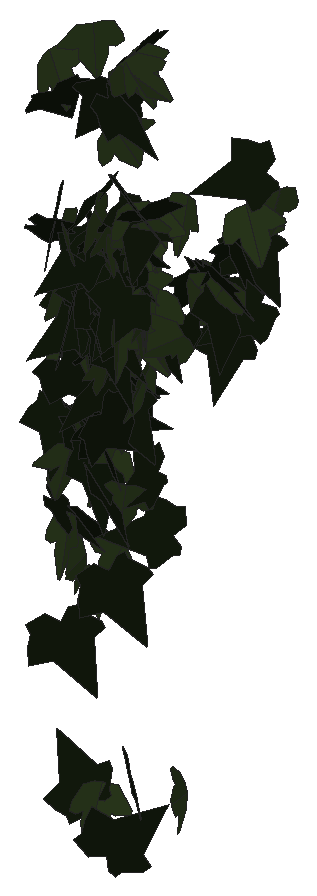
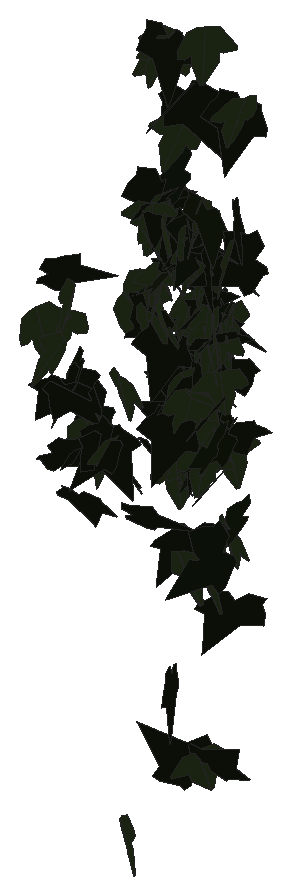
# SketchUp Ruby script. Lengths in inches.
U = 1.inch
M = Sketchup.active_model
def pt(a) = Geom::Point3d.new(a.map { |v| v * U })
def face(e, loops, mat)
  f = e.add_face(loops[0].map { |a| pt(a) })
  loops[1..].each { |l| e.add_face(l.map { |a| pt(a) }).erase! }
  f.material = f.back_material = mat if mat
  f
end
# faces: each face lists its corners as indices into pts; further lists are holes
def faces(e, pts, list, mat = nil) = list.each { |f| face(e, (f[0].is_a?(Array) ? f : [f]).map { |l| l.map { |i| pts[i] } }, mat) }
# xy, xz, yz: faces in a plane at the given z, y or x. An outline is a flat list of corners, or four numbers for a rectangle; further outlines are holes
def ring(l) = l.size == 4 ? [[l[0], l[1]], [l[2], l[1]], [l[2], l[3]], [l[0], l[3]]] : l.each_slice(2).to_a
def flat(e, list, mat, &to3) = list.each { |f| face(e, (f[0].is_a?(Array) ? f : [f]).map { |l| ring(l).map { |u, v| to3.(u, v) } }, mat) }
def xy(e, z, list, mat = nil) = flat(e, list, mat) { |x, y| [x, y, z] }
def xz(e, y, list, mat = nil) = flat(e, list, mat) { |x, z| [x, y, z] }
def yz(e, x, list, mat = nil) = flat(e, list, mat) { |y, z| [x, y, z] }
def lines(e, pts, list) = list.each { |a, b| e.add_line(pt(pts[a]), pt(pts[b])) }
# prism: a flat outline (further loops are holes) pulled along v
def prism(e, loops, v, mat = nil)
  f = face(e, loops, mat); d = Geom::Vector3d.new(v.map { |x| x * U })
  f.pushpull(f.normal.samedirection?(d) ? d.length : -d.length)
end
def box(e, o, s, mat = nil) = prism(e, [[o, [o[0] + s[0], o[1], o[2]], [o[0] + s[0], o[1] + s[1], o[2]], [o[0], o[1] + s[1], o[2]]]], [0, 0, s[2]], mat)
def at(x, y, z, deg = 0) = Geom::Transformation.translation(pt([x, y, z])) * Geom::Transformation.rotation(ORIGIN, Z_AXIS, deg.degrees)
def axes(o, x, y, z) = Geom::Transformation.new([*x, 0, *y, 0, *z, 0, *pt(o).to_a, 1])
def part(name) = M.definitions.add(name)
# library, detail: a bought-in or finely detailed component or shape, given as its bounding box
def library(name, o, s) = part(name).tap { |d| box(d.entities, o, s) }
def detail(e, o, s) = box(e.add_group.entities, o, s)
def put(e, d, t, mat = nil) = e.add_instance(d, t).tap { |i| i.material = mat if mat }
def group(e, t, mat = nil) = e.add_group.tap { |g| g.transformation = t; g.material = mat if mat }.entities
root = M.entities
M.materials.add("efeu1").color = [18, 25, 13]
M.materials.add("efeu2").color = [43, 57, 29]
c1 = part("ivyleaf_9")
p = [[1.54,2.16,1.25],[1.36,2.04,1.19],[-0.21,0.99,0.68],[-0.71,1.11,0.82],[-0.85,0.86,0.67],[-0.8,0.17,0.21],
  [-0.9,-0.01,0.1],[-0.67,-0.16,-0.02],[-0.08,-0.08,-0.05],[-0.03,-0.6,-0.4],[0.65,-0.88,-0.66],[0.83,-0.6,-0.49],
  [1.29,-0.42,-0.43],[1.8125,-0.07,-0.26],[1.21,0.44,0.15]]
faces(c1.entities,p,[[0,1,2,3,4,5,6,7,8,9,10,11,12,13,14]],"efeu1")
c2 = part("ivyleaf_10")
p = [[0,0.5,-0.03],[-0.0625,2.02,-0.43],[-0.19,2.01,-0.46],[-0.54,1.05,-0.29],[-0.52,0.625,-0.18],[-0.83,0.76,-0.28],
  [-1.16,0.64,-0.33],[-1.15,0.33,-0.24],[-0.77,-0.39,0.02],[-0.3,-0.51,0.16],[0.04,-0.48,0.23],[-0.02,2.01,-0.4375],
  [-0.06,2.01,-0.43],[0.04,-0.49,0.23],[0.67,-0.49,0.14],[1.38,0.36,-0.2],[1.375,0.51,-0.24],[0.81,0.65,-0.19],
  [0.62,0.59,-0.15],[0.6,1.09,-0.28],[0.5,1.23,-0.31]]
faces(c2.entities,p,[[0,1,2,3,4,5,6,7,8,9,10],[11,12,0,13,14,15,16,17,18,19,20]],"efeu2")
put(root,c1,axes([565.39,131.8,220.8125],[0.83802,-0.38885,-0.28194],[-0.1596,0.30932,-0.90101],[0.45302,0.8283,0.20411]))
put(root,c1,axes([565.19,131.24,232.89],[0.89104,0.08996,0.39688],[0.38144,0.14832,-0.88998],[-0.14182,0.96409,0.09988]))
put(root,c2,axes([565.66,139.23,230.36],[0.8859,-0.31674,0.10492],[0.10472,-0.01868,-0.94065],[0.3168,0.89189,0.01756]))
put(root,c2,axes([565.6875,131.4,240.08],[0.14938,0.96069,0.23258],[-0.00135,0.23542,-0.97155],[-0.98844,0.14487,0.03648]))
put(root,c2,axes([565.79,132.5,227.57],[0.61609,0.68863,-0.07239],[-0.08852,-0.01777,-0.92243],[-0.68675,0.62007,0.05396]))
put(root,c1,axes([565.35,133.52,225],[0.66113,-0.63323,0.0891],[0.06131,-0.0648,-0.91546],[0.63653,0.66395,-0.00436]))
put(root,c1,axes([565.79,131.85,224.875],[-0.50138,-0.7549,-0.20222],[0.13854,0.1506,-0.90569],[0.76914,-0.51922,0.03131]))
put(root,c1,axes([566.3125,139.5,227.53],[0.02633,0.74002,-0.55639],[-0.19435,-0.53979,-0.72715],[-0.90522,0.13742,0.13993]))
put(root,c2,axes([565.85,131.64,230.13],[0.23134,-0.92137,-0.0694],[0.23513,0.12789,-0.91412],[0.89357,0.20489,0.25851]))
put(root,c1,axes([565.45,133.04,219.62],[1.10906,-0.06823,0.04669],[0.0468,0.00039,-1.11115],[0.06816,1.11004,0.00326]))
put(root,c2,axes([566.0625,132.56,230.17],[0.3828,-0.85358,-0.16599],[0.00986,0.18561,-0.93173],[0.86951,0.37368,0.08364]))
put(root,c2,axes([566.08,132.49,229.6],[-0.87235,-0.34319,-0.15132],[0.14182,0.05284,-0.93743],[0.34722,-0.8838,0.00272]))
put(root,c2,axes([565.85,131.85,219.91],[0.87494,-0.39676,0.27622],[0.24314,-0.13251,-0.9605],[0.41785,0.90789,-0.01948]))
put(root,c1,axes([566.01,132.79,229.5],[-0.4877,-0.79464,-0.1327],[0.1525,0.06126,-0.92731],[0.79108,-0.5017,0.09695]))
put(root,c1,axes([565.7,133.05,223.02],[0.35096,-0.85963,-0.00658],[0.03008,0.01938,-0.92785],[0.85913,0.35049,0.03517]))
put(root,c2,axes([566.3,131.45,233.01],[-0.50537,0.74211,0.40736],[-0.25236,0.32079,-0.89749],[-0.80807,-0.5643,0.02552]))
put(root,c2,axes([566.26,132.27,224.74],[-0.32315,0.76023,0.42336],[-0.18241,0.3824,-0.8259],[-0.85083,-0.37072,0.01627]))
put(root,c1,axes([566.3,130.59,239.39],[0.35852,0.92403,-0.00446],[0.00246,-0.00573,-0.99114],[-0.92404,0.3585,-0.00437]))
put(root,c2,axes([566.15,139.51,227.28],[-0.11661,0.93037,0.21226],[-0.03849,0.20908,-0.93757],[-0.9535,-0.12223,0.01189]))
put(root,c1,axes([566.02,131.3,234.48],[-0.42055,0.14549,-0.8766],[0.80426,-0.35005,-0.44395],[-0.37783,-0.90706,0.03072]))
put(root,c1,axes([566.87,137.78,225.45],[-0.1541,0.45417,0.79811],[-0.45206,0.66689,-0.46678],[-0.7993,-0.46473,0.11013]))
put(root,c1,axes([566.92,131.92,208.59],[-0.95813,-0.20161,-0.2108],[-0.20468,-0.05099,0.97908],[-0.20782,0.97972,0.00758]))
put(root,c1,axes([565.86,132.18,224.74],[0.9116,-0.15725,-0.03229],[-0.02068,0.06961,-0.92277],[0.15919,0.90951,0.06504]))
put(root,c2,axes([566.5,131.22,223.54],[-0.32914,-0.89291,0.23218],[0.01638,-0.25213,-0.94641],[0.92245,-0.31412,0.09965]))
put(root,c1,axes([566.05,139.76,227.68],[0.91534,0.02089,-0.13093],[-0.13075,-0.00935,-0.91556],[-0.022,0.92461,-0.0063]))
put(root,c2,axes([566.47,132.9,223.89],[-0.6777,-0.63529,-0.08735],[0.14232,-0.02508,-0.92175],[0.62528,-0.68285,0.11512]))
put(root,c1,axes([566.07,133.1,225.92],[0.21747,-0.89595,0.07704],[0.00318,-0.07849,-0.92184],[0.89925,0.21695,-0.01537]))
put(root,c1,axes([565.98,132.46,230.02],[0.47589,-0.82238,0.09023],[0.08451,-0.05523,-0.94907],[0.82299,0.48121,0.04528]))
put(root,c1,axes([566.3,131.08,216.12],[-0.17993,-0.67367,-0.8148],[0.17166,0.79693,-0.6968],[1.0432,-0.24733,-0.02587]))
put(root,c2,axes([566.8,132.46,230.1],[-0.78296,0.47162,0.20492],[-0.16485,0.12339,-0.91381],[-0.48707,-0.79987,-0.02014]))
put(root,c2,axes([566.35,132.11,218.53],[-0.26436,0.12261,0.94128],[0.55951,-0.76918,0.25733],[0.7668,0.60353,0.13674]))
put(root,c2,axes([566.8,132.13,229.01],[0.44381,-0.8263,-0.21183],[-0.11083,0.18091,-0.93787],[0.84579,0.45729,-0.01174]))
put(root,c1,axes([567.17,131.34,229.5],[-0.92217,-0.08295,0.1596],[-0.15457,-0.06083,-0.92474],[0.09197,-0.9339,0.04606]))
put(root,c1,axes([567.2,132.06,232.8],[0.18837,0.06026,-0.95069],[-0.95203,0.04526,-0.18577],[0.03278,0.96811,0.06787]))
put(root,c1,axes([566.61,131.46,230.21],[-0.44575,0.22398,-0.81419],[0.72404,-0.37242,-0.49884],[-0.43457,-0.85024,0.00402]))
put(root,c2,axes([566.8,133.375,226.52],[-0.63785,-0.62642,-0.23611],[0.14828,0.18583,-0.89358],[0.65281,-0.65427,-0.02774]))
put(root,c1,axes([566.33,131.93,224.16],[0.49627,-0.78109,0.08696],[0.0379,-0.07894,-0.92535],[0.785,0.49761,-0.0103]))
put(root,c1,axes([567.21,131.92,224.875],[0.33929,-0.52183,0.748],[-0.44607,0.60117,0.62174],[-0.79551,-0.55966,-0.0296]))
put(root,c1,axes([567.41,131.38,232.46],[-0.95596,-0.01075,0.11059],[-0.11063,0.00256,-0.95602],[0.01038,-0.96234,-0.00377]))
put(root,c1,axes([566.46,131.01,227.53],[-0.05682,-0.24632,-0.93817],[0.34316,0.87389,-0.25023],[0.90724,-0.34598,0.03589]))
put(root,c2,axes([567.125,131.99,217.74],[0.76798,-0.43627,-0.30648],[-0.26771,0.14923,-0.88325],[0.46108,0.8133,-0.00234]))
put(root,c2,axes([566.35,132.93,225.96],[-0.18724,-0.03178,-0.91314],[0.88821,0.21231,-0.18952],[0.21432,-0.90764,-0.01236]))
put(root,c1,axes([567.46,131.42,234.47],[-0.16691,0.89382,0.39563],[-0.17047,0.36859,-0.90464],[-0.96249,-0.22029,0.09162]))
put(root,c2,axes([566.45,131.73,228.74],[0.57995,-0.26114,0.70926],[0.69397,-0.17015,-0.63011],[0.2994,0.90024,0.08665]))
put(root,c2,axes([567.25,133.1875,218.66],[0.83583,-0.19406,-0.40644],[-0.36271,0.21792,-0.84995],[0.26701,0.90351,0.11771]))
put(root,c1,axes([567.04,133.96,225.55],[0.71553,0.5567,-0.18553],[-0.17237,-0.08027,-0.90563],[-0.56092,0.73482,0.04163]))
put(root,c1,axes([566.78,131.63,227.16],[0.68483,0.62,0.54441],[0.35418,0.4181,-0.92169],[-0.74521,0.76848,0.06224]))
put(root,c2,axes([567.56,139.24,227.53],[-0.78835,-0.30923,0.46934],[-0.37524,-0.31233,-0.83609],[0.41844,-0.86269,0.13447]))
put(root,c1,axes([567.1,140.29,224.96],[-0.71676,-0.47023,-0.42279],[0.44048,0.08724,-0.84379],[0.45369,-0.82758,0.15128]))
put(root,c2,axes([567.51,131.82,232.33],[-0.78982,0.38087,0.39228],[-0.35862,0.15937,-0.87679],[-0.41272,-0.86735,0.01115]))
put(root,c1,axes([567.26,132.19,230.65],[-0.44296,-0.84214,-0.07989],[0.01795,0.08081,-0.95128],[0.84573,-0.44279,-0.02166]))
put(root,c2,axes([567.48,132.9,226.92],[-0.32095,-0.84965,0.21537],[0.08216,-0.25751,-0.89344],[0.87266,-0.28824,0.16332]))
put(root,c2,axes([567.39,132,208.74],[0.51552,0.7927,-0.31086],[-0.15467,-0.27017,-0.94544],[-0.83731,0.53796,-0.01675]))
put(root,c2,axes([567.87,136.34,207.04],[0.46536,-0.46379,-0.75999],[-0.45344,0.61453,-0.65267],[0.7662,0.64536,0.07533]))
put(root,c2,axes([567.73,131.66,229.4],[-0.92019,-0.18524,0.08099],[-0.06927,-0.06571,-0.93728],[0.18993,-0.9214,0.05056]))
put(root,c2,axes([567.31,132.11,232.21],[0.89663,-0.22558,0.30391],[0.29945,-0.05509,-0.92438],[0.23146,0.94512,0.01865]))
put(root,c1,axes([567.84,131.67,224.07],[0.55245,0.01098,-0.77637],[-0.77388,0.08519,-0.54947],[0.06307,0.94905,0.05831]))
put(root,c2,axes([567.6875,132.35,223.18],[0.34521,0.71969,-0.48793],[-0.24953,-0.4209,-0.79736],[-0.83293,0.42437,0.03665]))
put(root,c1,axes([567.74,131.46,233.36],[0.26963,0.86857,0.37033],[0.0819,0.36217,-0.90906],[-0.94066,0.28049,0.027]))
put(root,c1,axes([567.28,138.7,228.41],[0.95299,-0.02334,-0.11756],[-0.11729,0.01243,-0.95323],[0.02468,0.96013,0.00949]))
put(root,c1,axes([567.29,131.9,230.11],[0.33727,-0.90199,-0.17381],[0.01853,0.1918,-0.95938],[0.91839,0.32738,0.08318]))
put(root,c1,axes([568.11,131.51,227.09],[-0.92702,0.10042,-0.11636],[0.1099,-0.06422,-0.93102],[-0.10744,-0.93209,0.05161]))
put(root,c2,axes([567.76,132.18,230.5],[-0.19009,0.90219,0.19635],[-0.07992,0.18364,-0.92115],[-0.91984,-0.2024,0.03946]))
put(root,c1,axes([567.53,139.47,226.78],[-0.05133,-0.95699,0.09048],[-0.01544,-0.08977,-0.9583],[0.96113,-0.05255,-0.01056]))
put(root,c1,axes([567.41,131.77,223.42],[0.16389,-1.02315,0.03667],[0.00226,-0.03678,-1.03618],[1.0238,0.16386,-0.00359]))
put(root,c2,axes([567.91,132.15,233.4],[0.11209,-0.94137,-0.19562],[-0.01993,0.19463,-0.94802],[0.96128,0.1138,0.00316]))
put(root,c2,axes([567.82,131.26,234.29],[0.21558,-0.79613,-0.5806],[0.11009,0.61008,-0.79566],[0.97918,0.10668,0.21728]))
put(root,c1,axes([567.79,132.27,232.625],[-0.48684,-0.8272,-0.06062],[0.05761,0.03639,-0.95933],[0.82741,-0.48925,0.03113]))
put(root,c1,axes([568.18,131.47,225.59],[-0.17538,0.8742,-0.61157],[0.14173,-0.5952,-0.89144],[-1.05743,-0.22476,-0.01805]))
put(root,c2,axes([567.94,131,242.34],[-0.61203,-0.79543,-0.0282],[0.12839,-0.06355,-0.99376],[0.78551,-0.60937,0.14046]))
put(root,c1,axes([567.125,132.84,226.62],[0.48863,-0.29121,0.74554],[0.64016,-0.38214,-0.56883],[0.48045,0.80533,-0.00033]))
put(root,c1,axes([568.3,139.58,229.66],[-0.23664,0.61176,-0.66923],[-0.02184,-0.69529,-0.62787],[-0.90645,-0.14296,0.18984]))
put(root,c1,axes([568.35,140.38,226.63],[-0.70675,-0.49822,0.42464],[-0.36112,-0.22451,-0.86443],[0.54603,-0.79336,-0.02205]))
put(root,c1,axes([568.44,131.45,239.71],[0.28981,0.43572,-0.848],[-0.48052,-0.69875,-0.52326],[-0.82345,0.56111,0.00689]))
put(root,c2,axes([567.5,132.81,225.11],[0.3572,-0.1859,0.84769],[0.75064,-0.39386,-0.40267],[0.43553,0.83129,-0.00122]))
put(root,c2,axes([568.18,131.55,228.09],[0.05379,-0.96605,0.06532],[0.02232,-0.06416,-0.96736],[0.96799,0.05516,0.01867]))
put(root,c2,axes([568.14,131.95,232.86],[-0.3168,0.86538,0.28397],[-0.13312,0.25344,-0.92084],[-0.901,-0.34172,0.0362]))
put(root,c1,axes([567.6,131.84,222.6],[0.53729,-0.80259,0.13286],[0.05747,-0.12138,-0.96563],[0.81148,0.54,-0.01958]))
put(root,c1,axes([567.42,132.84,224.93],[0.43552,-0.17995,0.81101],[0.74204,-0.32743,-0.47113],[0.37349,0.86035,-0.00967]))
put(root,c1,axes([568.4,132.78,228.62],[0.30154,0.88396,0.08357],[0.0451,0.07289,-0.93378],[-0.88675,0.3043,-0.01907]))
put(root,c2,axes([568.7,131.98,222.27],[-0.77961,-0.48598,0.17593],[-0.14576,-0.09874,-0.91865],[0.49587,-0.79309,0.00656]))
put(root,c1,axes([568.54,138.66,229.94],[0.68362,-0.26828,-0.63],[-0.56206,0.28861,-0.7328],[0.3911,0.88371,0.04807]))
put(root,c1,axes([568.35,131.47,218.86],[-0.01662,-0.77044,-0.77265],[0.03305,0.77203,-0.77053],[1.09063,-0.03513,0.01157]))
put(root,c1,axes([568.32,139.875,229.57],[-0.19184,-0.5819,-0.70819],[0.40744,0.59398,-0.59842],[0.82105,-0.43072,0.1315]))
put(root,c2,axes([568.85,138.83,233.3],[-0.67331,0.66108,0.08074],[-0.05794,0.05623,-0.94359],[-0.66346,-0.6758,0.00047]))
put(root,c1,axes([568.46,131.2,229.875],[0.56862,-0.66423,-0.43717],[-0.20917,0.39358,-0.87005],[0.76719,0.59962,0.08681]))
put(root,c1,axes([569.47,132.27,232.25],[-0.47098,0.58512,0.59344],[-0.34392,0.48444,-0.7506],[-0.75911,-0.58251,-0.02813]))
put(root,c2,axes([568.77,131.375,238.09],[0.46658,0.71175,0.52826],[-0.06516,0.6229,-0.78172],[-0.88396,0.32977,0.33645]))
put(root,c1,axes([568.37,131.93,226.22],[-0.12241,-0.57909,-0.75326],[0.52472,0.59196,-0.54035],[0.79209,-0.48163,0.24155]))
put(root,c1,axes([569.625,133.44,220.15],[-0.74222,0.15003,0.58821],[-0.60534,-0.11353,-0.73489],[-0.04534,-0.94021,0.1826]))
put(root,c1,axes([568.41,131.29,228.95],[0.40801,-0.8839,0.00025],[0.04288,0.01952,-0.97238],[0.88286,0.40755,0.04711]))
put(root,c1,axes([568.4,132.61,232.01],[0.62373,-0.70236,-0.12914],[0.03977,0.20536,-0.92481],[0.71302,0.60295,0.16455]))
put(root,c2,axes([568.91,132.25,233.52],[0.39912,-0.86014,0.1705],[0.0972,-0.14278,-0.94783],[0.87148,0.40986,0.02762]))
put(root,c1,axes([568.92,130.34,226.43],[0.14354,-0.32176,-1.03633],[-0.49912,0.90864,-0.35124],[0.96353,0.51861,-0.02757]))
put(root,c2,axes([569.0625,139.41,230.92],[-0.06243,0.46055,0.81864],[-0.2125,0.79225,-0.46191],[-0.91494,-0.21543,0.05143]))
put(root,c1,axes([568.25,132.3,232.75],[0.3994,-0.2927,0.82257],[0.65593,-0.49641,-0.49513],[0.57624,0.76794,-0.00653]))
put(root,c1,axes([569.52,132.7,223.12],[-0.91189,0.24865,0.00545],[-0.00571,-0.00023,-0.94518],[-0.24864,-0.9119,0.00173]))
put(root,c2,axes([569.01,131.28,229.78],[-0.12349,0.80902,-0.56806],[0.10828,-0.55796,-0.81817],[-0.98259,-0.16316,-0.01876]))
put(root,c1,axes([568.79,130.9,239.72],[0.63406,-0.63454,-0.47128],[-0.15717,0.49089,-0.87241],[0.77462,0.619,0.20875]))
put(root,c2,axes([569.23,132.57,227.18],[-0.17949,0.58583,-0.72328],[-0.13653,-0.74521,-0.56971],[-0.9207,-0.0037,0.22549]))
put(root,c2,axes([568.8,132.625,229.17],[0.38476,-0.56527,-0.65372],[0.37471,-0.5357,0.68377],[-0.77876,-0.53704,0.00602]))
put(root,c1,axes([569.41,131.3125,231.28],[-0.81356,-0.48363,-0.08834],[0.07053,0.05422,-0.9464],[0.48654,-0.81655,-0.01052]))
put(root,c1,axes([568.7,130.91,207.19],[-0.29765,0.04063,1.04046],[1.03717,-0.08423,0.29999],[0.09218,1.07892,-0.01576]))
put(root,c1,axes([569.63,131.33,241.91],[-0.05865,0.99871,0.08408],[0.0038,0.08445,-1.00039],[-1.00224,-0.05813,-0.00872]))
put(root,c2,axes([569.22,132.19,231.35],[0.24669,0.87462,0.26365],[-0.02708,0.27998,-0.90345],[-0.9131,0.22799,0.09802]))
put(root,c2,axes([568.71,132.64,228.8],[0.49908,-0.035,0.80259],[0.79637,0.14587,-0.48885],[-0.1057,0.93379,0.10645]))
put(root,c1,axes([568.875,131.31,235.89],[0.9027,-0.4291,-0.02418],[-0.0256,0.00248,-0.99946],[0.42902,0.90302,-0.00875]))
put(root,c2,axes([569.53,132.14,233.76],[-0.33135,-0.90238,0.10754],[0.01201,-0.1188,-0.95989],[0.90869,-0.32748,0.0519]))
put(root,c2,axes([569.32,131.65,234.59],[0.29186,0.91319,-0.1306],[-0.0393,-0.12455,-0.9587],[-0.92165,0.2945,-0.00048]))
put(root,c2,axes([569.24,133.03,229.43],[0.89546,-0.25647,0.11415],[0.15173,0.12112,-0.91813],[0.23619,0.89454,0.15704]))
put(root,c2,axes([569.54,132.15,230.43],[0.21818,-0.8252,-0.39831],[-0.01375,0.40645,-0.84959],[0.9162,0.20261,0.0821]))
put(root,c1,axes([569.91,130.72,211.07],[0.32857,0.05784,-0.91194],[-0.90155,0.17845,-0.31351],[0.14891,0.95276,0.11408]))
put(root,c1,axes([570.07,138.46,233.73],[-0.65126,-0.30049,0.65721],[-0.58217,-0.306,-0.7168],[0.42813,-0.87317,0.02503]))
put(root,c2,axes([569.38,132.16,230.73],[-0.42565,0.68254,-0.49002],[0.17051,-0.46772,-0.79958],[-0.82275,-0.45005,0.0878]))
put(root,c2,axes([569.55,131.89,233.91],[-0.74734,-0.56666,-0.24156],[0.23365,0.09064,-0.93551],[0.56997,-0.78017,0.06677]))
put(root,c1,axes([569.45,132.15,234.54],[-0.26707,-0.92883,-0.00992],[0.00877,0.0078,-0.96644],[0.92884,-0.26714,0.00627]))
put(root,c1,axes([569.8,131.53,235.02],[0.31748,0.91527,-0.10994],[-0.10719,-0.07884,-0.96586],[-0.91559,0.3266,0.07495]))
put(root,c2,axes([569.83,132.51,230.8],[-0.94713,-0.05365,0.0742],[-0.05466,-0.28729,-0.90549],[0.07346,-0.90556,0.28288]))
put(root,c1,axes([569.22,132.75,229.75],[-0.2887,-0.15655,-0.88325],[0.7617,0.44727,-0.32825],[0.47376,-0.81451,-0.01049]))
put(root,c2,axes([569.88,139.56,232.1],[-0.34229,-0.90405,0.17763],[-0.02048,-0.18198,-0.96566],[0.92111,-0.34,0.04454]))
put(root,c2,axes([569.58,132.33,234.18],[0.80286,0.50413,0.0797],[0.05568,0.06115,-0.94776],[-0.50734,0.80449,0.0221]))
put(root,c2,axes([569.55,138.26,231.7],[0.68902,0.63524,0.26075],[0.17014,0.19993,-0.93667],[-0.66526,0.70906,0.03051]))
put(root,c2,axes([569.85,131.28,241.56],[0.03197,0.96101,0.29051],[-0.01607,0.29111,-0.96123],[-1.00384,0.02594,0.02464]))
put(root,c2,axes([570.71,132.44,229.45],[-0.4833,-0.23982,0.78297],[-0.69767,-0.35542,-0.53951],[0.42874,-0.84871,0.00468]))
put(root,c2,axes([569.81,130.86,241.42],[-0.649,-0.33875,-0.68806],[0.60854,0.32111,-0.73209],[0.46675,-0.88967,-0.00225]))
